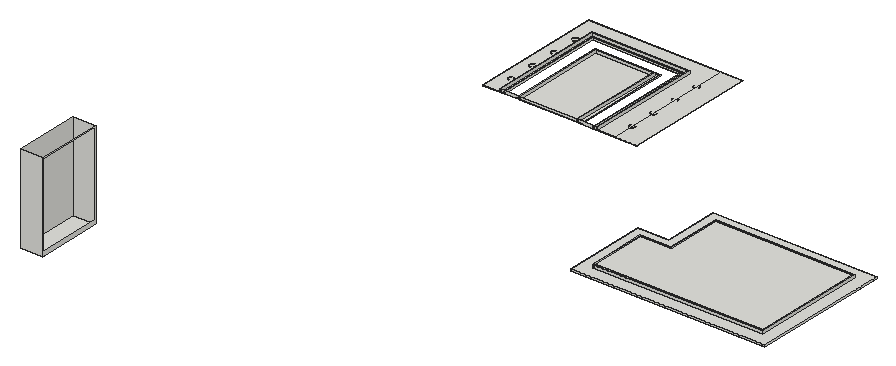
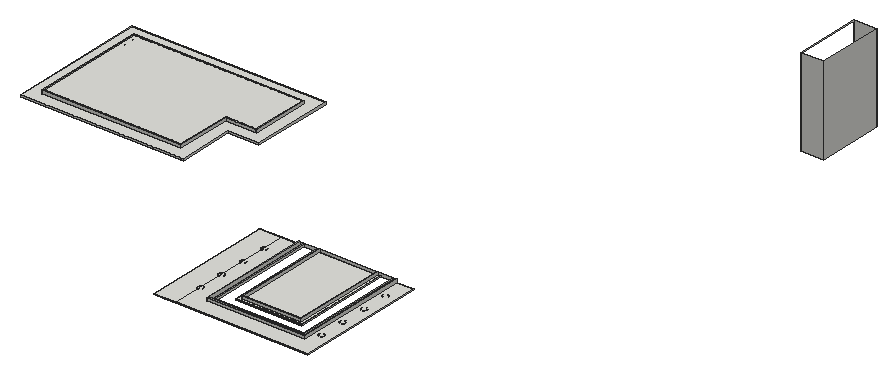
# SketchUp Ruby script. Lengths in inches.
U = 1.inch
M = Sketchup.active_model
def pt(a) = Geom::Point3d.new(a.map { |v| v * U })
def face(e, loops, mat)
  f = e.add_face(loops[0].map { |a| pt(a) })
  loops[1..].each { |l| e.add_face(l.map { |a| pt(a) }).erase! }
  f.material = f.back_material = mat if mat
  f
end
# faces: each face lists its corners as indices into pts; further lists are holes
def faces(e, pts, list, mat = nil) = list.each { |f| face(e, (f[0].is_a?(Array) ? f : [f]).map { |l| l.map { |i| pts[i] } }, mat) }
# xy, xz, yz: faces in a plane at the given z, y or x. An outline is a flat list of corners, or four numbers for a rectangle; further outlines are holes
def ring(l) = l.size == 4 ? [[l[0], l[1]], [l[2], l[1]], [l[2], l[3]], [l[0], l[3]]] : l.each_slice(2).to_a
def flat(e, list, mat, &to3) = list.each { |f| face(e, (f[0].is_a?(Array) ? f : [f]).map { |l| ring(l).map { |u, v| to3.(u, v) } }, mat) }
def xy(e, z, list, mat = nil) = flat(e, list, mat) { |x, y| [x, y, z] }
def xz(e, y, list, mat = nil) = flat(e, list, mat) { |x, z| [x, y, z] }
def yz(e, x, list, mat = nil) = flat(e, list, mat) { |y, z| [x, y, z] }
def lines(e, pts, list) = list.each { |a, b| e.add_line(pt(pts[a]), pt(pts[b])) }
# prism: a flat outline (further loops are holes) pulled along v
def prism(e, loops, v, mat = nil)
  f = face(e, loops, mat); d = Geom::Vector3d.new(v.map { |x| x * U })
  f.pushpull(f.normal.samedirection?(d) ? d.length : -d.length)
end
def box(e, o, s, mat = nil) = prism(e, [[o, [o[0] + s[0], o[1], o[2]], [o[0] + s[0], o[1] + s[1], o[2]], [o[0], o[1] + s[1], o[2]]]], [0, 0, s[2]], mat)
def at(x, y, z, deg = 0) = Geom::Transformation.translation(pt([x, y, z])) * Geom::Transformation.rotation(ORIGIN, Z_AXIS, deg.degrees)
def axes(o, x, y, z) = Geom::Transformation.new([*x, 0, *y, 0, *z, 0, *pt(o).to_a, 1])
def part(name) = M.definitions.add(name)
# library, detail: a bought-in or finely detailed component or shape, given as its bounding box
def library(name, o, s) = part(name).tap { |d| box(d.entities, o, s) }
def detail(e, o, s) = box(e.add_group.entities, o, s)
def put(e, d, t, mat = nil) = e.add_instance(d, t).tap { |i| i.material = mat if mat }
def group(e, t, mat = nil) = e.add_group.tap { |g| g.transformation = t; g.material = mat if mat }.entities
root = M.entities
xy(root,-0.08,[[675.99,527.85,675.7,527.86,675.2,527.88,674.45,528.11,673.79,528.52,673.26,529.09,672.89,529.78,672.71,530.55,672.74,531.33,672.97,532.08,673.38,532.74,673.95,533.28,674.65,533.65,675.41,533.82,675.7,533.8125,676.19,533.8,676.94,533.57,677.6,533.15,678.14,532.58,678.51,531.89,678.68,531.125,678.66,530.34,678.43,529.59,678.01,528.93,677.44,528.4,676.75,528.03],[807.7,527.85,806.95,527.88,806.2,528.11,805.54,528.52,805.01,529.09,804.64,529.78,804.46,530.55,804.49,531.33,804.72,532.08,805.13,532.74,805.7,533.28,806.4,533.65,807.16,533.82,807.45,533.8125,807.7,533.8,807.94,533.8,808.69,533.57,809.35,533.15,809.89,532.58,810.26,531.89,810.43,531.125,810.41,530.34,810.18,529.59,809.76,528.93,809.19,528.4,808.5,528.03,807.74,527.85],[675.95,556.85,675.2,556.88,674.45,557.11,673.79,557.52,673.26,558.09,672.89,558.78,672.71,559.55,672.74,560.33,672.97,561.08,673.38,561.74,673.95,562.28,674.65,562.65,675.41,562.82,675.7,562.8125,675.95,562.8,676.19,562.8,676.94,562.57,677.6,562.15,678.14,561.58,678.51,560.89,678.68,560.125,678.66,559.34,678.43,558.59,678.01,557.93,677.44,557.4,676.75,557.03,675.99,556.85],[807.7,556.85,806.95,556.88,806.2,557.11,805.54,557.52,805.01,558.09,804.64,558.78,804.46,559.55,804.49,560.33,804.72,561.08,805.13,561.74,805.7,562.28,806.4,562.65,807.16,562.82,807.45,562.8125,807.7,562.8,807.94,562.8,808.69,562.57,809.35,562.15,809.89,561.58,810.26,560.89,810.43,560.125,810.41,559.34,810.18,558.59,809.76,557.93,809.19,557.4,808.5,557.03,807.74,556.85],[675.95,585.85,675.7,585.86,675.41,585.87,675.2,585.88,674.45,586.11,673.79,586.52,673.26,587.09,672.89,587.78,672.71,588.55,672.74,589.33,672.97,590.08,673.38,590.74,673.95,591.28,674.65,591.65,675.41,591.82,675.7,591.8125,675.95,591.8,676.19,591.8,676.94,591.57,677.6,591.15,678.14,590.58,678.51,589.89,678.68,589.125,678.66,588.34,678.43,587.59,678.01,586.93,677.44,586.4,676.75,586.03,675.99,585.85],
  [807.7,585.85,807.45,585.86,807.16,585.87,806.95,585.88,806.2,586.11,805.54,586.52,805.01,587.09,804.64,587.78,804.46,588.55,804.49,589.33,804.72,590.08,805.13,590.74,805.7,591.28,806.4,591.65,807.16,591.82,807.45,591.8125,807.7,591.8,807.94,591.8,808.69,591.57,809.35,591.15,809.89,590.58,810.26,589.89,810.43,589.125,810.41,588.34,810.18,587.59,809.76,586.93,809.19,586.4,808.5,586.03,807.74,585.85]])
xy(root,0,[[533.16,41.91,557.16,113.91],[[663.7,506.84,663.7,650.84,795.7,650.84,795.7,506.84,783.7,506.84,783.7,626.84,687.7,626.84,687.7,506.84],[675.95,556.85,675.99,556.85,676.75,557.03,677.44,557.4,678.01,557.93,678.43,558.59,678.66,559.34,678.68,560.125,678.51,560.89,678.14,561.58,677.6,562.15,676.94,562.57,676.19,562.8,675.95,562.8,675.7,562.8125,675.41,562.82,674.65,562.65,673.95,562.28,673.38,561.74,672.97,561.08,672.74,560.33,672.71,559.55,672.89,558.78,673.26,558.09,673.79,557.52,674.45,557.11,675.2,556.88],[675.99,527.85,676.75,528.03,677.44,528.4,678.01,528.93,678.43,529.59,678.66,530.34,678.68,531.125,678.51,531.89,678.14,532.58,677.6,533.15,676.94,533.57,676.19,533.8,675.7,533.8125,675.41,533.82,674.65,533.65,673.95,533.28,673.38,532.74,672.97,532.08,672.74,531.33,672.71,530.55,672.89,529.78,673.26,529.09,673.79,528.52,674.45,528.11,675.2,527.88,675.7,527.86],[675.95,614.85,675.99,614.85,676.75,615.03,677.44,615.4,678.01,615.93,678.43,616.59,678.66,617.34,678.68,618.125,678.51,618.89,678.14,619.58,677.6,620.15,676.94,620.57,676.19,620.8,675.95,620.8,675.7,620.8125,675.41,620.82,674.65,620.65,673.95,620.28,673.38,619.74,672.97,619.08,672.74,618.33,672.71,617.55,672.89,616.78,673.26,616.09,673.79,615.52,674.45,615.11,675.2,614.88,675.41,614.87,675.7,614.86],[675.95,585.85,675.99,585.85,676.75,586.03,677.44,586.4,678.01,586.93,678.43,587.59,678.66,588.34,678.68,589.125,678.51,589.89,678.14,590.58,677.6,591.15,676.94,591.57,676.19,591.8,675.95,591.8,675.7,591.8125,675.41,591.82,674.65,591.65,673.95,591.28,673.38,590.74,672.97,590.08,672.74,589.33,672.71,588.55,672.89,587.78,673.26,587.09,673.79,586.52,674.45,586.11,675.2,585.88,675.41,585.87,675.7,585.86]],[699.7,506.84,771.7,614.84],[[795.7,506.84,819.7,650.84],[807.7,556.85,807.74,556.85,808.5,557.03,809.19,557.4,809.76,557.93,810.18,558.59,810.41,559.34,810.43,560.125,810.26,560.89,809.89,561.58,809.35,562.15,808.69,562.57,807.94,562.8,807.7,562.8,807.45,562.8125,807.16,562.82,806.4,562.65,805.7,562.28,805.13,561.74,804.72,561.08,804.49,560.33,804.46,559.55,804.64,558.78,805.01,558.09,805.54,557.52,806.2,557.11,806.95,556.88],[807.7,585.85,807.74,585.85,808.5,586.03,809.19,586.4,809.76,586.93,810.18,587.59,810.41,588.34,810.43,589.125,810.26,589.89,809.89,590.58,809.35,591.15,808.69,591.57,807.94,591.8,807.7,591.8,807.45,591.8125,807.16,591.82,806.4,591.65,805.7,591.28,805.13,590.74,804.72,590.08,804.49,589.33,804.46,588.55,804.64,587.78,805.01,587.09,805.54,586.52,806.2,586.11,806.95,585.88,807.16,585.87,807.45,585.86],[807.7,614.85,807.74,614.85,808.5,615.03,809.19,615.4,809.76,615.93,810.18,616.59,810.41,617.34,810.43,618.125,810.26,618.89,809.89,619.58,809.35,620.15,808.69,620.57,807.94,620.8,807.7,620.8,807.45,620.8125,807.16,620.82,806.4,620.65,805.7,620.28,805.13,619.74,804.72,619.08,804.49,618.33,804.46,617.55,804.64,616.78,805.01,616.09,805.54,615.52,806.2,615.11,806.95,614.88,807.16,614.87,807.45,614.86],[807.7,527.85,807.74,527.85,808.5,528.03,809.19,528.4,809.76,528.93,810.18,529.59,810.41,530.34,810.43,531.125,810.26,531.89,809.89,532.58,809.35,533.15,808.69,533.57,807.94,533.8,807.7,533.8,807.45,533.8125,807.16,533.82,806.4,533.65,805.7,533.28,805.13,532.74,804.72,532.08,804.49,531.33,804.46,530.55,804.64,529.78,805.01,529.09,805.54,528.52,806.2,528.11,806.95,527.88]],[819.7,506.84,831.7,650.84]])
xy(root,0.04,[[807.7,614.85,807.45,614.86,807.16,614.87,806.95,614.88,806.2,615.11,805.54,615.52,805.01,616.09,804.64,616.78,804.46,617.55,804.49,618.33,804.72,619.08,805.13,619.74,805.7,620.28,806.4,620.65,807.16,620.82,807.45,620.8125,807.7,620.8,807.94,620.8,808.69,620.57,809.35,620.15,809.89,619.58,810.26,618.89,810.43,618.125,810.41,617.34,810.18,616.59,809.76,615.93,809.19,615.4,808.5,615.03,807.74,614.85]])
xy(root,0.49,[[663.7,506.84,682.7,506.84,682.7,631.84,788.7,631.84,788.7,506.84,807.7,506.84,807.7,650.84,663.7,650.84],[683.7,506.84,686.7,506.84,686.7,627.84,784.7,627.84,784.7,506.84,787.7,506.84,787.7,630.84,683.7,630.84],[699.7,506.84,700.7,506.84,700.7,613.84,770.7,613.84,770.7,506.84,771.7,506.84,771.7,614.84,699.7,614.84],[700.7,506.84,703.7,506.84,703.7,610.84,767.7,610.84,767.7,506.84,770.7,506.84,770.7,613.84,700.7,613.84],[704.7,506.84,766.7,609.84],
  [807.7,506.84,831.7,650.84]])
xz(root,41.91,[[533.16,0,557.16,96]])
xz(root,113.91,[[533.16,0,557.16,96]])
xz(root,506.84,[[663.7,0,687.7,0,687.7,1.99,686.7,1.99,686.7,0.49,683.7,0.49,683.7,3.49,682.7,3.49,682.7,0.49,663.7,0.49],[687.7,0,699.7,0,699.7,0.49,703.7,0.49,703.7,3.49,683.7,3.49,683.7,0.49,686.7,0.49,686.7,1.99,687.7,1.99],[699.7,0,771.7,0,771.7,0.49,767.7,0.49,767.7,3.49,766.7,3.49,766.7,0.49,704.7,0.49,704.7,3.49,703.7,3.49,703.7,0.49,699.7,0.49],[771.7,0,783.7,0,783.7,1.99,784.7,1.99,784.7,0.49,787.7,0.49,787.7,3.49,767.7,3.49,767.7,0.49,771.7,0.49],[783.7,0,807.7,0,807.7,0.49,788.7,0.49,788.7,3.49,787.7,3.49,787.7,0.49,784.7,0.49,784.7,1.99,783.7,1.99],
  [807.7,0,831.7,0.49],[704.7,0.49,766.7,3.49]])
xz(root,527.85,[[807.7,-0.08,807.74,0]])
xz(root,533.8,[[807.7,-0.08,807.94,0]])
xz(root,556.85,[[675.95,-0.08,675.99,0],[807.7,-0.08,807.74,0]])
xz(root,562.8,[[675.95,-0.08,676.19,0],[807.7,-0.08,807.94,0]])
xz(root,585.85,[[675.95,-0.08,675.99,0],[807.7,-0.08,807.74,0]])
xz(root,591.8,[[675.95,-0.08,676.19,0],[807.7,-0.08,807.94,0]])
xz(root,609.84,[[704.7,0.49,766.7,3.49]])
xz(root,610.84,[[703.7,0.49,767.7,3.49]])
xz(root,614.84,[[699.7,0,771.7,0.49]])
xz(root,614.85,[[675.95,0,675.99,0.04],[807.7,0,807.74,0.04]])
xz(root,620.8,[[675.95,0,676.19,0.04],[807.7,0,807.94,0.04]])
xz(root,626.84,[[687.7,0,783.7,1.99]])
xz(root,627.84,[[686.7,0.49,784.7,1.99]])
xz(root,630.84,[[683.7,0.49,787.7,3.49]])
xz(root,631.84,[[682.7,0.49,788.7,3.49]])
xz(root,650.84,[[663.7,0,807.7,0.49],[807.7,0,831.7,0.49]])
yz(root,533.16,[[41.91,0,113.91,96]])
yz(root,557.16,[[[41.91,0,113.91,96],[42.66,4,113.16,95.25]]])
yz(root,663.7,[[506.84,0,650.84,0.49]])
yz(root,682.7,[[506.84,0.49,631.84,3.49]])
yz(root,683.7,[[506.84,0.49,630.84,3.49]])
yz(root,686.7,[[506.84,0.49,627.84,1.99]])
yz(root,687.7,[[506.84,0,626.84,1.99]])
yz(root,699.7,[[506.84,0,614.84,0.49]])
yz(root,703.7,[[506.84,0.49,610.84,3.49]])
yz(root,704.7,[[506.84,0.49,609.84,3.49]])
yz(root,766.7,[[506.84,0.49,609.84,3.49]])
yz(root,767.7,[[506.84,0.49,610.84,3.49]])
yz(root,771.7,[[506.84,0,614.84,0.49]])
yz(root,783.7,[[506.84,0,626.84,1.99]])
yz(root,784.7,[[506.84,0.49,627.84,1.99]])
yz(root,787.7,[[506.84,0.49,630.84,3.49]])
yz(root,788.7,[[506.84,0.49,631.84,3.49]])
yz(root,831.7,[[506.84,0,650.84,0.49]])
p = [[675.2,527.88,0],[674.45,528.11,0],[674.45,528.11,-0.08],[675.2,527.88,-0.08],[675.7,527.86,0],[675.7,527.86,-0.08],
  [675.99,527.85,0],[675.99,527.85,-0.08],[676.75,528.03,0],[676.75,528.03,-0.08],[806.95,527.88,0],[806.2,528.11,0],
  [806.2,528.11,-0.08],[806.95,527.88,-0.08],[807.45,527.86,0],[807.45,527.86,-0.08],[807.7,527.85,0],[807.7,527.85,-0.08],
  [808.5,528.03,0],[807.74,527.85,0],[807.74,527.85,-0.08],[808.5,528.03,-0.08],[677.44,528.4,0],[677.44,528.4,-0.08],
  [809.19,528.4,0],[809.19,528.4,-0.08],[673.79,528.52,0],[673.79,528.52,-0.08],[805.54,528.52,0],[805.54,528.52,-0.08],
  [678.01,528.93,0],[678.01,528.93,-0.08],[809.76,528.93,0],[809.76,528.93,-0.08],[673.26,529.09,0],[673.26,529.09,-0.08],
  [805.01,529.09,0],[805.01,529.09,-0.08],[678.43,529.59,0],[678.43,529.59,-0.08],[810.18,529.59,0],[810.18,529.59,-0.08],
  [672.89,529.78,0],[672.89,529.78,-0.08],[804.64,529.78,0],[804.64,529.78,-0.08],[678.66,530.34,0],[678.66,530.34,-0.08],
  [810.41,530.34,0],[810.41,530.34,-0.08],[672.71,530.55,0],[672.71,530.55,-0.08],[804.46,530.55,0],[804.46,530.55,-0.08],
  [678.68,531.125,0],[678.68,531.125,-0.08],[810.43,531.125,0],[810.43,531.125,-0.08],[672.74,531.33,0],[672.74,531.33,-0.08],
  [804.49,531.33,0],[804.49,531.33,-0.08],[678.51,531.89,0],[678.51,531.89,-0.08],[810.26,531.89,0],[810.26,531.89,-0.08],
  [672.97,532.08,0],[672.97,532.08,-0.08],[804.72,532.08,0],[804.72,532.08,-0.08],[678.14,532.58,0],[678.14,532.58,-0.08],
  [809.89,532.58,0],[809.89,532.58,-0.08],[673.38,532.74,0],[673.38,532.74,-0.08],[805.13,532.74,0],[805.13,532.74,-0.08],
  [677.6,533.15,0],[677.6,533.15,-0.08],[809.35,533.15,0],[809.35,533.15,-0.08],[673.95,533.28,0],[673.95,533.28,-0.08],
  [805.7,533.28,0],[805.7,533.28,-0.08],[676.94,533.57,0],[676.94,533.57,-0.08],[808.69,533.57,0],[808.69,533.57,-0.08],
  [674.65,533.65,0],[674.65,533.65,-0.08],[806.4,533.65,0],[806.4,533.65,-0.08],[675.41,533.82,0],[675.41,533.82,-0.08],
  [676.19,533.8,0],[676.19,533.8,-0.08],[807.16,533.82,0],[807.16,533.82,-0.08],[807.94,533.8,0],[807.94,533.8,-0.08],
  [675.7,533.8125,0],[675.7,533.8125,-0.08],[807.45,533.8125,0],[807.45,533.8125,-0.08],[807.7,533.8,0],[807.7,533.8,-0.08],
  [675.2,556.88,0],[674.45,557.11,0],[674.45,557.11,-0.08],[675.2,556.88,-0.08],[675.7,556.86,0],[675.7,556.86,-0.08],
  [675.95,556.85,0],[675.95,556.85,-0.08],[676.75,557.03,0],[675.99,556.85,0],[675.99,556.85,-0.08],[676.75,557.03,-0.08],
  [806.95,556.88,0],[806.2,557.11,0],[806.2,557.11,-0.08],[806.95,556.88,-0.08],[807.45,556.86,0],[807.45,556.86,-0.08],
  [807.7,556.85,0],[807.7,556.85,-0.08],[808.5,557.03,0],[807.74,556.85,0],[807.74,556.85,-0.08],[808.5,557.03,-0.08],
  [677.44,557.4,0],[677.44,557.4,-0.08],[809.19,557.4,0],[809.19,557.4,-0.08],[673.79,557.52,0],[673.79,557.52,-0.08],
  [805.54,557.52,0],[805.54,557.52,-0.08],[678.01,557.93,0],[678.01,557.93,-0.08],[809.76,557.93,0],[809.76,557.93,-0.08],
  [673.26,558.09,0],[673.26,558.09,-0.08],[805.01,558.09,0],[805.01,558.09,-0.08],[678.43,558.59,0],[678.43,558.59,-0.08],
  [810.18,558.59,0],[810.18,558.59,-0.08],[672.89,558.78,0],[672.89,558.78,-0.08],[804.64,558.78,0],[804.64,558.78,-0.08],
  [678.66,559.34,0],[678.66,559.34,-0.08],[810.41,559.34,0],[810.41,559.34,-0.08],[672.71,559.55,0],[672.71,559.55,-0.08],
  [804.46,559.55,0],[804.46,559.55,-0.08],[678.68,560.125,0],[678.68,560.125,-0.08],[810.43,560.125,0],[810.43,560.125,-0.08],
  [672.74,560.33,0],[672.74,560.33,-0.08],[804.49,560.33,0],[804.49,560.33,-0.08],[678.51,560.89,0],[678.51,560.89,-0.08],
  [810.26,560.89,0],[810.26,560.89,-0.08],[672.97,561.08,0],[672.97,561.08,-0.08],[804.72,561.08,0],[804.72,561.08,-0.08],
  [678.14,561.58,0],[678.14,561.58,-0.08],[809.89,561.58,0],[809.89,561.58,-0.08],[673.38,561.74,0],[673.38,561.74,-0.08],
  [805.13,561.74,0],[805.13,561.74,-0.08],[677.6,562.15,0],[677.6,562.15,-0.08],[809.35,562.15,0],[809.35,562.15,-0.08],
  [673.95,562.28,0],[673.95,562.28,-0.08],[805.7,562.28,0],[805.7,562.28,-0.08],[676.94,562.57,0],[676.94,562.57,-0.08],
  [808.69,562.57,0],[808.69,562.57,-0.08],[674.65,562.65,0],[674.65,562.65,-0.08],[806.4,562.65,0],[806.4,562.65,-0.08],
  [675.41,562.82,0],[675.41,562.82,-0.08],[676.19,562.8,0],[676.19,562.8,-0.08],[807.16,562.82,0],[807.16,562.82,-0.08],
  [807.94,562.8,0],[807.94,562.8,-0.08],[675.7,562.8125,0],[675.7,562.8125,-0.08],[675.95,562.8,0],[675.95,562.8,-0.08],
  [807.45,562.8125,0],[807.45,562.8125,-0.08],[807.7,562.8,0],[807.7,562.8,-0.08],[675.2,585.88,0],[674.45,586.11,0],
  [674.45,586.11,-0.08],[675.2,585.88,-0.08],[675.41,585.87,0],[675.41,585.87,-0.08],[675.7,585.86,0],[675.7,585.86,-0.08],
  [675.95,585.85,0],[675.95,585.85,-0.08],[676.75,586.03,0],[675.99,585.85,0],[675.99,585.85,-0.08],[676.75,586.03,-0.08],
  [806.95,585.88,0],[806.2,586.11,0],[806.2,586.11,-0.08],[806.95,585.88,-0.08],[807.16,585.87,0],[807.16,585.87,-0.08],
  [807.45,585.86,0],[807.45,585.86,-0.08],[807.7,585.85,0],[807.7,585.85,-0.08],[808.5,586.03,0],[807.74,585.85,0],
  [807.74,585.85,-0.08],[808.5,586.03,-0.08],[677.44,586.4,0],[677.44,586.4,-0.08],[809.19,586.4,0],[809.19,586.4,-0.08],
  [673.79,586.52,0],[673.79,586.52,-0.08],[805.54,586.52,0],[805.54,586.52,-0.08],[678.01,586.93,0],[678.01,586.93,-0.08],
  [809.76,586.93,0],[809.76,586.93,-0.08],[673.26,587.09,0],[673.26,587.09,-0.08],[805.01,587.09,0],[805.01,587.09,-0.08],
  [678.43,587.59,0],[678.43,587.59,-0.08],[810.18,587.59,0],[810.18,587.59,-0.08],[672.89,587.78,0],[672.89,587.78,-0.08],
  [804.64,587.78,0],[804.64,587.78,-0.08],[678.66,588.34,0],[678.66,588.34,-0.08],[810.41,588.34,0],[810.41,588.34,-0.08],
  [672.71,588.55,0],[672.71,588.55,-0.08],[804.46,588.55,0],[804.46,588.55,-0.08],[678.68,589.125,0],[678.68,589.125,-0.08],
  [810.43,589.125,0],[810.43,589.125,-0.08],[672.74,589.33,0],[672.74,589.33,-0.08],[804.49,589.33,0],[804.49,589.33,-0.08],
  [678.51,589.89,0],[678.51,589.89,-0.08],[810.26,589.89,0],[810.26,589.89,-0.08],[672.97,590.08,0],[672.97,590.08,-0.08],
  [804.72,590.08,0],[804.72,590.08,-0.08],[678.14,590.58,0],[678.14,590.58,-0.08],[809.89,590.58,0],[809.89,590.58,-0.08],
  [673.38,590.74,0],[673.38,590.74,-0.08],[805.13,590.74,0],[805.13,590.74,-0.08],[677.6,591.15,0],[677.6,591.15,-0.08],
  [809.35,591.15,0],[809.35,591.15,-0.08],[673.95,591.28,0],[673.95,591.28,-0.08],[805.7,591.28,0],[805.7,591.28,-0.08],
  [676.94,591.57,0],[676.94,591.57,-0.08],[808.69,591.57,0],[808.69,591.57,-0.08],[674.65,591.65,0],[674.65,591.65,-0.08],
  [806.4,591.65,0],[806.4,591.65,-0.08],[675.41,591.82,0],[675.41,591.82,-0.08],[676.19,591.8,0],[676.19,591.8,-0.08],
  [807.16,591.82,0],[807.16,591.82,-0.08],[807.94,591.8,0],[807.94,591.8,-0.08],[675.7,591.8125,0],[675.7,591.8125,-0.08],
  [675.95,591.8,0],[675.95,591.8,-0.08],[807.45,591.8125,0],[807.45,591.8125,-0.08],[807.7,591.8,0],[807.7,591.8,-0.08],
  [675.2,614.88,0],[674.45,615.11,0],[674.45,615.11,0.04],[675.2,614.88,0.04],[675.41,614.87,0],[675.41,614.87,0.04],
  [675.7,614.86,0],[675.7,614.86,0.04],[675.95,614.85,0],[675.95,614.85,0.04],[676.75,615.03,0],[675.99,614.85,0],
  [675.99,614.85,0.04],[676.75,615.03,0.04],[806.95,614.88,0],[806.2,615.11,0],[806.2,615.11,0.04],[806.95,614.88,0.04],
  [807.16,614.87,0],[807.16,614.87,0.04],[807.45,614.86,0],[807.45,614.86,0.04],[807.7,614.85,0],[807.7,614.85,0.04],
  [808.5,615.03,0],[807.74,614.85,0],[807.74,614.85,0.04],[808.5,615.03,0.04],[677.44,615.4,0],[677.44,615.4,0.04],
  [809.19,615.4,0],[809.19,615.4,0.04],[673.79,615.52,0],[673.79,615.52,0.04],[805.54,615.52,0],[805.54,615.52,0.04],
  [678.01,615.93,0],[678.01,615.93,0.04],[809.76,615.93,0],[809.76,615.93,0.04],[673.26,616.09,0],[673.26,616.09,0.04],
  [805.01,616.09,0],[805.01,616.09,0.04],[678.43,616.59,0],[678.43,616.59,0.04],[810.18,616.59,0],[810.18,616.59,0.04],
  [672.89,616.78,0],[672.89,616.78,0.04],[804.64,616.78,0],[804.64,616.78,0.04],[678.66,617.34,0],[678.66,617.34,0.04],
  [810.41,617.34,0],[810.41,617.34,0.04],[672.71,617.55,0],[672.71,617.55,0.04],[804.46,617.55,0],[804.46,617.55,0.04],
  [678.68,618.125,0],[678.68,618.125,0.04],[810.43,618.125,0],[810.43,618.125,0.04],[672.74,618.33,0],[672.74,618.33,0.04],
  [804.49,618.33,0],[804.49,618.33,0.04],[678.51,618.89,0],[678.51,618.89,0.04],[810.26,618.89,0],[810.26,618.89,0.04],
  [672.97,619.08,0],[672.97,619.08,0.04],[804.72,619.08,0],[804.72,619.08,0.04],[678.14,619.58,0],[678.14,619.58,0.04],
  [809.89,619.58,0],[809.89,619.58,0.04],[673.38,619.74,0],[673.38,619.74,0.04],[805.13,619.74,0],[805.13,619.74,0.04],
  [677.6,620.15,0],[677.6,620.15,0.04],[809.35,620.15,0],[809.35,620.15,0.04],[673.95,620.28,0],[673.95,620.28,0.04],
  [805.7,620.28,0],[805.7,620.28,0.04],[676.94,620.57,0],[676.94,620.57,0.04],[808.69,620.57,0],[808.69,620.57,0.04],
  [674.65,620.65,0],[674.65,620.65,0.04],[806.4,620.65,0],[806.4,620.65,0.04],[675.41,620.82,0],[675.41,620.82,0.04],
  [676.19,620.8,0],[676.19,620.8,0.04],[807.16,620.82,0],[807.16,620.82,0.04],[807.94,620.8,0],[807.94,620.8,0.04],
  [675.7,620.8125,0],[675.7,620.8125,0.04],[675.95,620.8,0],[675.95,620.8,0.04],[807.45,620.8125,0],[807.45,620.8125,0.04],
  [807.7,620.8,0],[807.7,620.8,0.04]]
faces(root,p,[[0,1,2,3],[4,0,3,5],[6,4,5,7],[8,6,7,9],[10,11,12,13],[14,10,13,15],[16,14,15,17],[18,19,20,21],
  [22,8,9,23],[24,18,21,25],[1,26,27,2],[11,28,29,12],[30,22,23,31],[32,24,25,33],[26,34,35,27],[28,36,37,29],
  [38,30,31,39],[40,32,33,41],[34,42,43,35],[36,44,45,37],[46,38,39,47],[48,40,41,49],[42,50,51,43],[44,52,53,45],
  [54,46,47,55],[56,48,49,57],[50,58,59,51],[52,60,61,53],[62,54,55,63],[64,56,57,65],[58,66,67,59],[60,68,69,61],
  [70,62,63,71],[72,64,65,73],[66,74,75,67],[68,76,77,69],[78,70,71,79],[80,72,73,81],[74,82,83,75],[76,84,85,77],
  [86,78,79,87],[88,80,81,89],[82,90,91,83],[84,92,93,85],[90,94,95,91],[96,86,87,97],[92,98,99,93],[100,88,89,101],
  [94,102,103,95],[102,96,97,103],[98,104,105,99],[104,106,107,105],[108,109,110,111],[112,108,111,113],[114,112,113,115],[116,117,118,119],
  [120,121,122,123],[124,120,123,125],[126,124,125,127],[128,129,130,131],[132,116,119,133],[134,128,131,135],[109,136,137,110],[121,138,139,122],
  [140,132,133,141],[142,134,135,143],[136,144,145,137],[138,146,147,139],[148,140,141,149],[150,142,143,151],[144,152,153,145],[146,154,155,147],
  [156,148,149,157],[158,150,151,159],[152,160,161,153],[154,162,163,155],[164,156,157,165],[166,158,159,167],[160,168,169,161],[162,170,171,163],
  [172,164,165,173],[174,166,167,175],[168,176,177,169],[170,178,179,171],[180,172,173,181],[182,174,175,183],[176,184,185,177],[178,186,187,179],
  [188,180,181,189],[190,182,183,191],[184,192,193,185],[186,194,195,187],[196,188,189,197],[198,190,191,199],[192,200,201,193],[194,202,203,195],
  [200,204,205,201],[206,196,197,207],[202,208,209,203],[210,198,199,211],[204,212,213,205],[212,214,215,213],[208,216,217,209],[216,218,219,217],
  [220,221,222,223],[224,220,223,225],[226,224,225,227],[228,226,227,229],[230,231,232,233],[234,235,236,237],[238,234,237,239],[240,238,239,241],
  [242,240,241,243],[244,245,246,247],[248,230,233,249],[250,244,247,251],[221,252,253,222],[235,254,255,236],[256,248,249,257],[258,250,251,259],
  [252,260,261,253],[254,262,263,255],[264,256,257,265],[266,258,259,267],[260,268,269,261],[262,270,271,263],[272,264,265,273],[274,266,267,275],
  [268,276,277,269],[270,278,279,271],[280,272,273,281],[282,274,275,283],[276,284,285,277],[278,286,287,279],[288,280,281,289],[290,282,283,291],
  [284,292,293,285],[286,294,295,287],[296,288,289,297],[298,290,291,299],[292,300,301,293],[294,302,303,295],[304,296,297,305],[306,298,299,307],
  [300,308,309,301],[302,310,311,303],[312,304,305,313],[314,306,307,315],[308,316,317,309],[310,318,319,311],[316,320,321,317],[322,312,313,323],
  [318,324,325,319],[326,314,315,327],[320,328,329,321],[328,330,331,329],[324,332,333,325],[332,334,335,333],[336,337,338,339],[340,336,339,341],
  [342,340,341,343],[344,342,343,345],[346,347,348,349],[350,351,352,353],[354,350,353,355],[356,354,355,357],[358,356,357,359],[360,361,362,363],
  [364,346,349,365],[366,360,363,367],[337,368,369,338],[351,370,371,352],[372,364,365,373],[374,366,367,375],[368,376,377,369],[370,378,379,371],
  [380,372,373,381],[382,374,375,383],[376,384,385,377],[378,386,387,379],[388,380,381,389],[390,382,383,391],[384,392,393,385],[386,394,395,387],
  [396,388,389,397],[398,390,391,399],[392,400,401,393],[394,402,403,395],[404,396,397,405],[406,398,399,407],[400,408,409,401],[402,410,411,403],
  [412,404,405,413],[414,406,407,415],[408,416,417,409],[410,418,419,411],[420,412,413,421],[422,414,415,423],[416,424,425,417],[418,426,427,419],
  [428,420,421,429],[430,422,423,431],[424,432,433,425],[426,434,435,427],[432,436,437,433],[438,428,429,439],[434,440,441,435],[442,430,431,443],
  [436,444,445,437],[444,446,447,445],[440,448,449,441],[448,450,451,449]])
g1 = group(root,at(923.03,303.02,0))
xy(g1,0,[[[0,0,0,90.79,33.46,90.79,33.46,151.42,210.87,151.42,210.87,0],[18,18,192.87,18,192.87,133.42,51.46,133.42,51.46,72.79,18,72.79]]])
xy(g1,2,[[[0,0,210.87,0,210.87,151.42,33.46,151.42,33.46,90.79,0,90.79],[13,13,13,77.79,46.46,77.79,46.46,138.42,197.87,138.42,197.87,13]],[[14,14,196.87,14,196.87,137.42,47.46,137.42,47.46,76.79,14,76.79],[17,17,17,73.79,50.46,73.79,50.46,134.42,193.87,134.42,193.87,17]]])
xy(g1,3.5,[[[17,17,193.87,17,193.87,134.42,50.46,134.42,50.46,73.79,17,73.79],[18,18,18,72.79,51.46,72.79,51.46,133.42,192.87,133.42,192.87,18]]])
xy(g1,5,[[[13,13,197.87,13,197.87,138.42,46.46,138.42,46.46,77.79,13,77.79],[14,14,14,76.79,47.46,76.79,47.46,137.42,196.87,137.42,196.87,14]],[14,14,196.87,14,196.87,137.42,47.46,137.42,47.46,76.79,14,76.79]])
xz(g1,0,[[0,0,210.87,2]])
xz(g1,13,[[13,2,197.87,5]])
xz(g1,14,[[14,2,196.87,5]])
xz(g1,17,[[17,2,193.87,3.5]])
xz(g1,18,[[18,0,192.87,3.5]])
xz(g1,72.79,[[18,0,51.46,3.5]])
xz(g1,73.79,[[17,2,50.46,3.5]])
xz(g1,76.79,[[14,2,47.46,5]])
xz(g1,77.79,[[13,2,46.46,5]])
xz(g1,90.79,[[0,0,33.46,2]])
xz(g1,133.42,[[51.46,0,192.87,3.5]])
xz(g1,134.42,[[50.46,2,193.87,3.5]])
xz(g1,137.42,[[47.46,2,196.87,5]])
xz(g1,138.42,[[46.46,2,197.87,5]])
xz(g1,151.42,[[33.46,0,210.87,2]])
yz(g1,0,[[0,0,90.79,2]])
yz(g1,13,[[13,2,77.79,5]])
yz(g1,14,[[14,2,76.79,5]])
yz(g1,17,[[17,2,73.79,3.5]])
yz(g1,18,[[18,0,72.79,3.5]])
yz(g1,33.46,[[90.79,0,151.42,2]])
yz(g1,46.46,[[77.79,2,138.42,5]])
yz(g1,47.46,[[76.79,2,137.42,5]])
yz(g1,50.46,[[73.79,2,134.42,3.5]])
yz(g1,51.46,[[72.79,0,133.42,3.5]])
yz(g1,192.87,[[18,0,133.42,3.5]])
yz(g1,193.87,[[17,2,134.42,3.5]])
yz(g1,196.87,[[14,2,137.42,5]])
yz(g1,197.87,[[13,2,138.42,5]])
yz(g1,210.87,[[0,0,151.42,2]])
